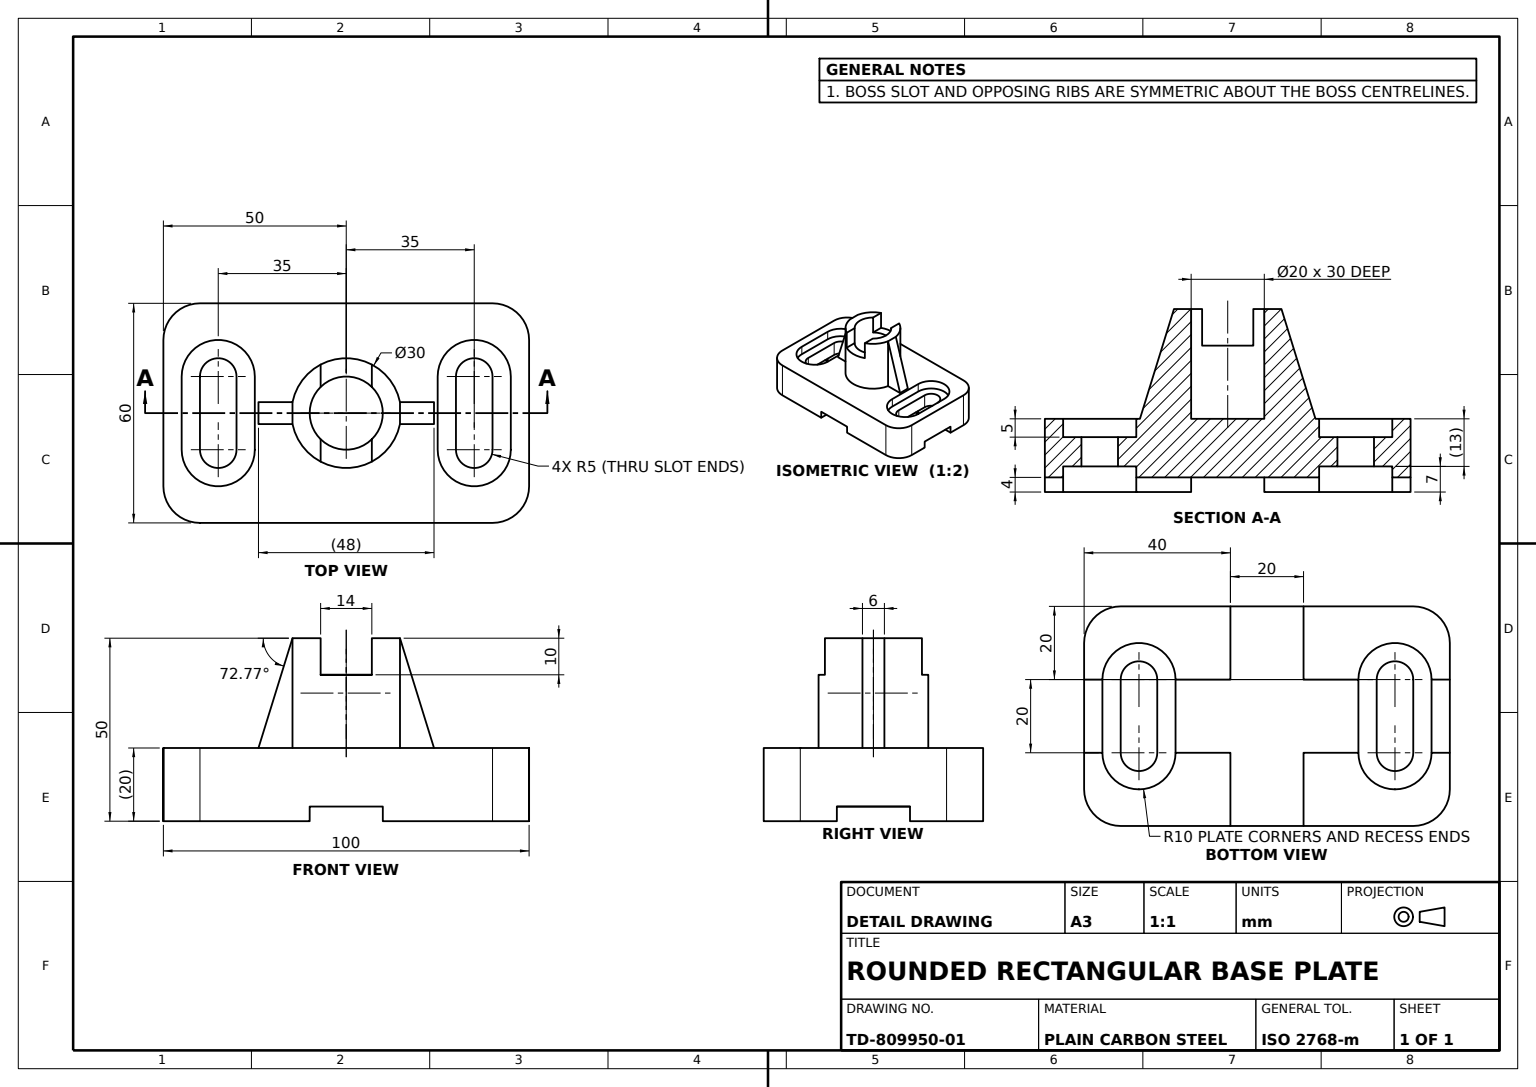
solid
v1 (40,7,-10)
v2 (30,7,-10)
e1 v1 v2 CIRCLE(AX(P(35,7,-10),D(0,1,0),D(-1,0,0)),5)
v3 (40,15,-10)
e2 v1 v3 LINE
v4 (30,15,-10)
e3 v4 v3 CIRCLE(AX(P(35,15,-10),D(0,-1,0),D(-1,0,0)),5)
e4 v2 v4 LINE
face CYL(AX(P(35,7,-10),D(0,1,0),D(-1,0,0)),5) rev [-e1 e2 -e3 -e4]
v5 (-50,0,20)
v6 (-50,0,10)
e5 v5 v6 LINE
v7 (-45,0,10)
e6 v6 v7 LINE
v8 (-25,0,10)
e7 v8 v7 CIRCLE(AX(P(-35,0,10),D(0,-1,0),D(0,0,1)),10)
v9 (-10,0,10)
e8 v8 v9 LINE
v10 (-10,0,30)
e9 v10 v9 LINE
v11 (-40,0,30)
e10 v11 v10 LINE
e11 v11 v5 CIRCLE(AX(P(-40,0,20),D(0,-1,0),D(0,0,1)),10)
face PLANE(AX(P(-10,0,30),D(0,1,0),D(0,0,1))) rev [e5 e6 -e7 e8 -e9 -e10 e11]
v12 (-10,4,-30)
v13 (10,4,-30)
e12 v12 v13 LINE
v14 (-10,0,-30)
e13 v14 v12 LINE
v15 (-40,0,-30)
e14 v15 v14 LINE
v16 (-40,20,-30)
e15 v16 v15 LINE
v17 (40,20,-30)
e16 v17 v16 LINE
v18 (40,0,-30)
e17 v17 v18 LINE
v19 (10,0,-30)
e18 v19 v18 LINE
e19 v13 v19 LINE
face PLANE(AX(P(0,0,-30),D(0,0,1),D(1,0,0))) rev [-e12 -e13 -e14 -e15 -e16 e17 -e18 -e19]
v20 (-45,4,10)
v21 (-45,4,-10)
e20 v20 v21 LINE
v22 (-45,7,-10)
e21 v22 v21 LINE
v23 (-45,7,10)
e22 v23 v22 LINE
e23 v23 v20 LINE
face PLANE(AX(P(-45,7,10),D(-1,0,0),D(0,0,1))) rev [e20 -e21 -e22 e23]
v24 (-10,4,10)
e24 v9 v24 LINE
v25 (-10,4,30)
e25 v25 v24 LINE
e26 v10 v25 LINE
face PLANE(AX(P(-10,4,30),D(-1,0,0),D(0,0,1))) rev [e24 -e25 -e26 e9]
v26 (-14.696938,50,-3)
v27 (-14.696938,50,3)
e27 v26 v27 LINE
v28 (-24,20,-3)
e28 v28 v26 LINE
v29 (-24,20,3)
e29 v29 v28 LINE
e30 v27 v29 LINE
face PLANE(AX(P(-24,20,-30),D(0.955129755,-0.296187696,0),D(0.296187696,0.955129755,0))) rev [-e27 -e28 -e29 -e30]
v30 (7,40,7.141428)
v31 (-7,40,7.141428)
e31 v30 v31 CIRCLE(AX(P(0,40,0),D(0,-1,0),D(0,0,-1)),10)
v32 (7,50,7.141428)
e32 v32 v30 LINE
v33 (10,50,0)
e33 v32 v33 CIRCLE(AX(P(0,50,0),D(0,1,0),D(-1,0,0)),10)
v34 (10,20,0)
e34 v33 v34 LINE
v35 (-10,20,0)
e35 v35 v34 CIRCLE(AX(P(0,20,0),D(0,1,0),D(-1,0,0)),10)
v36 (-10,50,0)
e36 v36 v35 LINE
v37 (-7,50,7.141428)
e37 v36 v37 CIRCLE(AX(P(0,50,0),D(0,1,0),D(-1,0,0)),10)
e38 v31 v37 LINE
face CYL(AX(P(0,50,0),D(0,-1,0),D(1,0,0)),10) rev [-e31 -e32 e33 e34 -e35 -e36 e37 -e38]
v38 (24,20,-3)
v39 (14.696938,20,-3)
e39 v38 v39 LINE
v40 (14.696938,50,-3)
e40 v39 v40 LINE
e41 v40 v38 LINE
face PLANE(AX(P(24,50,-3),D(0,0,1),D(0,-1,0))) rev [e39 e40 e41]
v41 (-7,50,13.266499)
e42 v37 v41 LINE
v42 (-7,50,-7.141428)
e43 v42 v36 CIRCLE(AX(P(0,50,0),D(0,1,0),D(-1,0,0)),10)
v43 (-7,50,-13.266499)
e44 v43 v42 LINE
e45 v43 v26 CIRCLE(AX(P(0,50,0),D(0,1,0),D(-1,0,0)),15)
e46 v27 v41 CIRCLE(AX(P(0,50,0),D(0,1,0),D(-1,0,0)),15)
face PLANE(AX(P(0,50,0),D(0,1,0),D(-1,0,0))) [-e42 -e37 -e43 -e44 e45 e27 e46]
v44 (-40,7,-10)
v45 (-40,7,10)
e47 v44 v45 LINE
v46 (-40,15,-10)
e48 v44 v46 LINE
v47 (-40,15,10)
e49 v46 v47 LINE
e50 v45 v47 LINE
face PLANE(AX(P(-40,7,10),D(-1,0,0),D(0,-1,0))) rev [-e47 e48 e49 -e50]
v48 (25,7,-10)
v49 (35,7,-20)
e51 v48 v49 CIRCLE(AX(P(35,7,-10),D(0,-1,0),D(0,0,-1)),10)
v50 (25,4,-10)
e52 v48 v50 LINE
v51 (25,0,-10)
e53 v50 v51 LINE
v52 (35,0,-20)
e54 v51 v52 CIRCLE(AX(P(35,0,-10),D(0,-1,0),D(0,0,-1)),10)
e55 v49 v52 LINE
face CYL(AX(P(35,7,-10),D(0,-1,0),D(0,0,-1)),10) rev [-e51 e52 e53 e54 -e55]
v53 (-50,4,10)
e56 v53 v20 LINE
v54 (-50,4,-10)
e57 v54 v53 LINE
e58 v54 v21 LINE
face PLANE(AX(P(-50,4,0),D(0,1,0),D(0,0,1))) rev [-e20 -e56 -e57 e58]
v55 (30,7,10)
e59 v2 v55 LINE
v56 (30,15,10)
e60 v56 v4 LINE
e61 v55 v56 LINE
face PLANE(AX(P(30,7,10),D(-1,0,0),D(0,0,1))) rev [-e59 e4 -e60 -e61]
v57 (-45,0,-10)
e62 v21 v57 LINE
v58 (-50,0,-10)
e63 v58 v54 LINE
e64 v58 v57 LINE
face PLANE(AX(P(-50,4,-10),D(0,0,-1),D(0,1,0))) rev [-e62 -e58 -e63 e64]
v59 (10,4,30)
e65 v25 v59 LINE
v60 (10,0,30)
e66 v59 v60 LINE
v61 (40,0,30)
e67 v60 v61 LINE
v62 (40,20,30)
e68 v62 v61 LINE
v63 (-40,20,30)
e69 v62 v63 LINE
e70 v63 v11 LINE
face PLANE(AX(P(0,0,30),D(0,0,1),D(1,0,0))) [e26 e65 e66 e67 -e68 e69 e70 e10]
v64 (25,15,-10)
v65 (25,20,-10)
e71 v64 v65 LINE
v66 (25,20,10)
e72 v65 v66 LINE
v67 (25,15,10)
e73 v67 v66 LINE
e74 v64 v67 LINE
face PLANE(AX(P(25,15,10),D(-1,0,0),D(0,-1,0))) rev [e71 e72 -e73 -e74]
v68 (-7,40,-13.266499)
v69 (-7,40,-7.141428)
e75 v68 v69 LINE
v70 (7,40,-7.141428)
e76 v69 v70 CIRCLE(AX(P(0,40,0),D(0,-1,0),D(0,0,-1)),10)
v71 (7,40,-13.266499)
e77 v71 v70 LINE
e78 v68 v71 CIRCLE(AX(P(0,40,0),D(0,-1,0),D(0,0,-1)),15)
face PLANE(AX(P(7,40,-30),D(0,-1,0),D(0,0,-1))) rev [e75 e76 -e77 -e78]
v72 (-25,7,-10)
v73 (-25,4,-10)
e79 v72 v73 LINE
v74 (-25,4,10)
e80 v73 v74 LINE
v75 (-25,7,10)
e81 v75 v74 LINE
e82 v72 v75 LINE
face PLANE(AX(P(-25,7,10),D(1,0,0),D(0,0,-1))) rev [e79 e80 -e81 -e82]
v76 (-30,7,10)
v77 (-30,7,-10)
e83 v76 v77 LINE
v78 (-30,15,10)
e84 v76 v78 LINE
v79 (-30,15,-10)
e85 v78 v79 LINE
e86 v77 v79 LINE
face PLANE(AX(P(-30,7,10),D(1,0,0),D(0,0,-1))) rev [-e83 e84 e85 -e86]
e87 v74 v8 LINE
e88 v74 v24 LINE
face PLANE(AX(P(-50,0,10),D(0,0,1),D(1,0,0))) rev [-e8 -e87 e88 -e24]
e89 v77 v44 CIRCLE(AX(P(-35,7,-10),D(0,1,0),D(1,0,0)),5)
e90 v45 v76 CIRCLE(AX(P(-35,7,10),D(0,1,0),D(1,0,0)),5)
v80 (-35,7,-20)
e91 v80 v72 CIRCLE(AX(P(-35,7,-10),D(0,-1,0),D(0,0,1)),10)
e92 v75 v23 CIRCLE(AX(P(-35,7,10),D(0,-1,0),D(0,0,1)),10)
e93 v22 v80 CIRCLE(AX(P(-35,7,-10),D(0,-1,0),D(0,0,1)),10)
face PLANE(AX(P(-35,7,10),D(0,1,0),D(0,0,1))) rev [e83 e89 e47 e90] [e91 e82 e92 e22 e93]
e94 v79 v46 CIRCLE(AX(P(-35,15,-10),D(0,1,0),D(1,0,0)),5)
face CYL(AX(P(-35,7,-10),D(0,1,0),D(-1,0,0)),5) rev [e86 e94 -e48 -e89]
v81 (10,0,-10)
v82 (10,4,-10)
e95 v81 v82 LINE
e96 v82 v13 LINE
e97 v81 v19 LINE
face PLANE(AX(P(10,4,30),D(1,0,0),D(0,0,-1))) rev [e95 e96 e19 -e97]
v83 (10,0,10)
v84 (25,0,10)
e98 v83 v84 LINE
v85 (45,0,10)
e99 v85 v84 CIRCLE(AX(P(35,0,10),D(0,-1,0),D(0,0,-1)),10)
v86 (50,0,10)
e100 v85 v86 LINE
v87 (50,0,20)
e101 v87 v86 LINE
e102 v87 v61 CIRCLE(AX(P(40,0,20),D(0,-1,0),D(0,0,1)),10)
e103 v60 v83 LINE
face PLANE(AX(P(10,0,30),D(0,1,0),D(0,0,1))) rev [e98 -e99 e100 -e101 e102 -e67 e103]
v88 (-10,0,-10)
e104 v88 v14 LINE
v89 (-25,0,-10)
e105 v89 v88 LINE
v90 (-35,0,-20)
e106 v90 v89 CIRCLE(AX(P(-35,0,-10),D(0,-1,0),D(0,0,1)),10)
e107 v57 v90 CIRCLE(AX(P(-35,0,-10),D(0,-1,0),D(0,0,1)),10)
v91 (-50,0,-20)
e108 v58 v91 LINE
e109 v91 v15 CIRCLE(AX(P(-40,0,-20),D(0,-1,0),D(0,0,1)),10)
face PLANE(AX(P(-10,0,30),D(0,1,0),D(0,0,1))) rev [e14 -e104 -e105 -e106 -e107 -e64 e108 e109]
v92 (50,0,-10)
v93 (50,0,-20)
e110 v92 v93 LINE
v94 (45,0,-10)
e111 v94 v92 LINE
e112 v52 v94 CIRCLE(AX(P(35,0,-10),D(0,-1,0),D(0,0,-1)),10)
e113 v81 v51 LINE
e114 v18 v93 CIRCLE(AX(P(40,0,-20),D(0,-1,0),D(0,0,1)),10)
face PLANE(AX(P(10,0,30),D(0,1,0),D(0,0,1))) rev [-e110 -e111 -e112 -e54 -e113 e97 e18 e114]
v95 (50,4,10)
e115 v95 v86 LINE
v96 (45,4,10)
e116 v96 v85 LINE
e117 v96 v95 LINE
face PLANE(AX(P(-50,0,10),D(0,0,1),D(1,0,0))) rev [e115 -e100 -e116 e117]
e118 v53 v6 LINE
v97 (-50,20,20)
e119 v5 v97 LINE
v98 (-50,20,-20)
e120 v97 v98 LINE
e121 v91 v98 LINE
face PLANE(AX(P(-50,0,30),D(1,0,0),D(0,0,-1))) rev [e57 e118 -e5 e119 e120 -e121 -e108 e63]
e122 v80 v90 LINE
face CYL(AX(P(-35,7,-10),D(0,-1,0),D(0,0,-1)),10) rev [e62 e107 -e122 -e93 e21]
v99 (50,20,-20)
e123 v93 v99 LINE
e124 v17 v99 CIRCLE(AX(P(40,20,-20),D(0,-1,0),D(-1,0,0)),10)
face CYL(AX(P(40,-40,-20),D(0,1,0),D(-1,0,0)),10) [-e123 -e114 -e17 e124]
v100 (7,50,13.266499)
v101 (14.696938,50,3)
e125 v100 v101 CIRCLE(AX(P(0,50,0),D(0,1,0),D(-1,0,0)),15)
v102 (7,40,13.266499)
e126 v100 v102 LINE
v103 (-7,40,13.266499)
e127 v102 v103 CIRCLE(AX(P(0,40,0),D(0,-1,0),D(0,0,-1)),15)
e128 v103 v41 LINE
v104 (-14.696938,20,3)
e129 v104 v27 LINE
v105 (14.696938,20,3)
e130 v104 v105 CIRCLE(AX(P(0,20,0),D(0,1,0),D(1,0,0)),15)
e131 v101 v105 LINE
face CYL(AX(P(0,50,0),D(0,-1,0),D(1,0,0)),15) [-e125 e126 e127 e128 -e46 -e129 e130 -e131]
v106 (25,4,10)
e132 v106 v50 LINE
v107 (25,7,10)
e133 v107 v48 LINE
e134 v107 v106 LINE
face PLANE(AX(P(25,7,10),D(-1,0,0),D(0,0,1))) rev [e132 -e52 -e133 e134]
v108 (40,7,10)
e135 v55 v108 CIRCLE(AX(P(35,7,10),D(0,1,0),D(-1,0,0)),5)
e136 v108 v1 LINE
v109 (45,7,-10)
e137 v49 v109 CIRCLE(AX(P(35,7,-10),D(0,-1,0),D(0,0,-1)),10)
v110 (45,7,10)
e138 v109 v110 LINE
e139 v110 v107 CIRCLE(AX(P(35,7,10),D(0,-1,0),D(0,0,-1)),10)
face PLANE(AX(P(35,7,10),D(0,-1,0),D(0,0,-1))) [e1 e59 e135 e136] [e137 e138 e139 e133 e51]
e140 v34 v35 CIRCLE(AX(P(0,20,0),D(0,1,0),D(-1,0,0)),10)
face PLANE(AX(P(50,20,30),D(0,-1,0),D(1,0,0))) rev [e35 e140]
v111 (-14.696938,20,-3)
e141 v111 v28 LINE
e142 v39 v111 CIRCLE(AX(P(0,20,0),D(0,1,0),D(1,0,0)),15)
v112 (24,20,3)
e143 v112 v38 LINE
e144 v112 v105 LINE
e145 v104 v29 LINE
v113 (45,20,10)
e146 v66 v113 CIRCLE(AX(P(35,20,10),D(0,1,0),D(-1,0,0)),10)
v114 (45,20,-10)
e147 v114 v65 CIRCLE(AX(P(35,20,-10),D(0,1,0),D(-1,0,0)),10)
e148 v113 v114 LINE
e149 v63 v97 CIRCLE(AX(P(-40,20,20),D(0,-1,0),D(-1,0,0)),10)
v115 (50,20,20)
e150 v115 v62 CIRCLE(AX(P(40,20,20),D(0,-1,0),D(1,0,0)),10)
e151 v115 v99 LINE
e152 v98 v16 CIRCLE(AX(P(-40,20,-20),D(0,-1,0),D(1,0,0)),10)
v116 (-45,20,-10)
v117 (-45,20,10)
e153 v116 v117 LINE
v118 (-25,20,-10)
e154 v118 v116 CIRCLE(AX(P(-35,20,-10),D(0,1,0),D(1,0,0)),10)
v119 (-25,20,10)
e155 v119 v118 LINE
e156 v117 v119 CIRCLE(AX(P(-35,20,10),D(0,1,0),D(1,0,0)),10)
face PLANE(AX(P(50,20,30),D(0,-1,0),D(1,0,0))) rev [e29 -e141 -e142 -e39 -e143 e144 -e130 e145] [-e146 -e72 -e147 -e148] [-e149 -e69 -e150 e151 -e124 e16 -e152 -e120] [-e153 -e154 -e155 -e156]
v120 (7,50,-13.266499)
v121 (7,50,-7.141428)
e157 v120 v121 LINE
e158 v71 v120 LINE
e159 v70 v121 LINE
face PLANE(AX(P(7,50,-30),D(1,0,0),D(0,1,0))) rev [-e157 -e158 e77 e159]
e160 v89 v73 LINE
face CYL(AX(P(-35,7,-10),D(0,-1,0),D(0,0,-1)),10) rev [-e91 e122 e106 e160 -e79]
e161 v47 v78 CIRCLE(AX(P(-35,15,10),D(0,1,0),D(1,0,0)),5)
face CYL(AX(P(-35,7,10),D(0,1,0),D(-1,0,0)),5) rev [e50 e161 -e84 -e90]
v122 (-45,15,-10)
v123 (-45,15,10)
e162 v122 v123 LINE
v124 (-25,15,10)
e163 v123 v124 CIRCLE(AX(P(-35,15,10),D(0,1,0),D(1,0,0)),10)
v125 (-25,15,-10)
e164 v124 v125 LINE
e165 v125 v122 CIRCLE(AX(P(-35,15,-10),D(0,1,0),D(1,0,0)),10)
face PLANE(AX(P(-35,15,10),D(0,-1,0),D(1,0,0))) rev [-e161 -e49 -e94 -e85] [e162 e163 e164 e165]
e166 v82 v50 LINE
face PLANE(AX(P(-50,4,-10),D(0,0,-1),D(0,1,0))) rev [-e95 e113 -e53 -e166]
face PLANE(AX(P(24,20,3),D(0,0,-1),D(0,1,0))) rev [-e145 e129 e30]
v126 (10,4,10)
e167 v59 v126 LINE
e168 v126 v83 LINE
face PLANE(AX(P(10,4,30),D(1,0,0),D(0,0,-1))) rev [-e66 e167 e168 -e103]
e169 v123 v117 LINE
e170 v124 v119 LINE
face CYL(AX(P(-35,15,10),D(0,1,0),D(-1,0,0)),10) rev [-e163 e169 e156 -e170]
e171 v43 v68 LINE
e172 v40 v120 CIRCLE(AX(P(0,50,0),D(0,1,0),D(-1,0,0)),15)
e173 v26 v111 LINE
face CYL(AX(P(0,50,0),D(0,-1,0),D(1,0,0)),15) [-e45 e171 e78 e158 -e172 -e40 e142 -e173]
e174 v126 v106 LINE
v127 (-10,4,-10)
e175 v73 v127 LINE
e176 v127 v12 LINE
face PLANE(AX(P(-10,4,30),D(0,1,0),D(0,0,1))) rev [e12 -e96 e166 -e132 -e174 -e167 -e65 e25 -e88 -e80 e175 e176]
v128 (45,15,-10)
e177 v128 v114 LINE
e178 v128 v64 CIRCLE(AX(P(35,15,-10),D(0,1,0),D(-1,0,0)),10)
face CYL(AX(P(35,15,-10),D(0,1,0),D(-1,0,0)),10) rev [e177 e147 -e71 -e178]
v129 (45,4,-10)
v130 (50,4,-10)
e179 v129 v130 LINE
e180 v94 v129 LINE
e181 v92 v130 LINE
face PLANE(AX(P(-50,4,-10),D(0,0,-1),D(0,1,0))) rev [-e179 -e180 e111 e181]
e182 v20 v7 LINE
face CYL(AX(P(-35,7,10),D(0,-1,0),D(0,0,-1)),10) rev [-e92 e81 e87 e7 -e182 -e23]
e183 v122 v116 LINE
e184 v125 v118 LINE
face CYL(AX(P(-35,15,-10),D(0,1,0),D(-1,0,0)),10) rev [e154 -e183 -e165 e184]
e185 v87 v115 LINE
face CYL(AX(P(40,-40,20),D(0,1,0),D(-1,0,0)),10) [e68 -e102 e185 e150]
e186 v109 v129 LINE
e187 v129 v96 LINE
e188 v110 v96 LINE
face PLANE(AX(P(45,7,10),D(1,0,0),D(0,0,-1))) rev [-e138 e186 e187 -e188]
v131 (40,15,10)
e189 v131 v56 CIRCLE(AX(P(35,15,10),D(0,-1,0),D(-1,0,0)),5)
e190 v3 v131 LINE
v132 (45,15,10)
e191 v67 v132 CIRCLE(AX(P(35,15,10),D(0,1,0),D(-1,0,0)),10)
e192 v132 v128 LINE
face PLANE(AX(P(35,15,10),D(0,1,0),D(-1,0,0))) [e189 e60 e3 e190] [e191 e192 e178 e74]
e193 v42 v69 LINE
e194 v33 v121 CIRCLE(AX(P(0,50,0),D(0,1,0),D(-1,0,0)),10)
face CYL(AX(P(0,50,0),D(0,-1,0),D(1,0,0)),10) rev [-e159 -e76 -e193 e43 e36 -e140 -e34 e194]
e195 v112 v101 LINE
face PLANE(AX(P(24,20,3),D(0,0,-1),D(0,1,0))) rev [e131 -e144 e195]
e196 v127 v88 LINE
face PLANE(AX(P(-50,4,-10),D(0,0,-1),D(0,1,0))) rev [e105 -e196 -e175 -e160]
e197 v84 v106 LINE
face PLANE(AX(P(-50,0,10),D(0,0,1),D(1,0,0))) rev [e174 -e197 -e98 -e168]
face PLANE(AX(P(-25,15,10),D(1,0,0),D(0,1,0))) rev [e170 e155 -e184 -e164]
face PLANE(AX(P(-7,40,-30),D(-1,0,0),D(0,-1,0))) rev [-e75 -e171 e44 e193]
e198 v130 v95 LINE
face PLANE(AX(P(-50,4,0),D(0,1,0),D(0,0,1))) rev [-e117 -e187 e179 e198]
e199 v108 v131 LINE
face CYL(AX(P(35,7,10),D(0,1,0),D(-1,0,0)),5) rev [-e199 -e135 e61 -e189]
face CYL(AX(P(35,7,-10),D(0,-1,0),D(0,0,-1)),10) rev [-e137 e55 e112 e180 -e186]
face PLANE(AX(P(-50,0,10),D(0,0,1),D(1,0,0))) rev [-e6 -e118 e56 e182]
e200 v132 v113 LINE
face CYL(AX(P(35,15,10),D(0,1,0),D(-1,0,0)),10) rev [e146 -e200 -e191 e73]
e201 v32 v100 LINE
e202 v40 v101 LINE
face PLANE(AX(P(0,50,0),D(0,1,0),D(-1,0,0))) [e201 e125 -e202 e172 e157 -e194 -e33]
face CYL(AX(P(-40,-40,-20),D(0,1,0),D(-1,0,0)),10) [e121 e152 e15 -e109]
e203 v30 v102 LINE
face PLANE(AX(P(7,50,-30),D(1,0,0),D(0,1,0))) rev [-e126 -e201 e32 e203]
face PLANE(AX(P(-45,15,10),D(-1,0,0),D(0,-1,0))) rev [e153 -e169 -e162 e183]
face CYL(AX(P(35,7,10),D(0,-1,0),D(0,0,-1)),10) rev [e197 -e134 -e139 e188 e116 e99]
face PLANE(AX(P(24,50,-3),D(0,0,1),D(0,-1,0))) rev [e141 e28 e173]
face PLANE(AX(P(40,7,10),D(1,0,0),D(0,1,0))) rev [-e2 -e136 e199 -e190]
face CYL(AX(P(-40,-40,20),D(0,1,0),D(-1,0,0)),10) [-e11 -e70 e149 -e119]
e204 v31 v103 LINE
face PLANE(AX(P(7,40,-30),D(0,-1,0),D(0,0,-1))) rev [e204 -e127 -e203 e31]
face PLANE(AX(P(-10,4,30),D(-1,0,0),D(0,0,1))) rev [e196 e104 e13 -e176]
face PLANE(AX(P(50,0,30),D(-1,0,0),D(0,0,1))) rev [e123 -e151 -e185 e101 -e115 -e198 -e181 e110]
face PLANE(AX(P(-7,40,-30),D(-1,0,0),D(0,-1,0))) rev [-e204 e38 e42 -e128]
face PLANE(AX(P(45,15,10),D(1,0,0),D(0,1,0))) rev [e148 -e177 -e192 e200]
face PLANE(AX(P(24,20,-30),D(-0.955129755,-0.296187696,0),D(0.296187696,-0.955129755,0))) rev [e143 -e41 e202 -e195]
